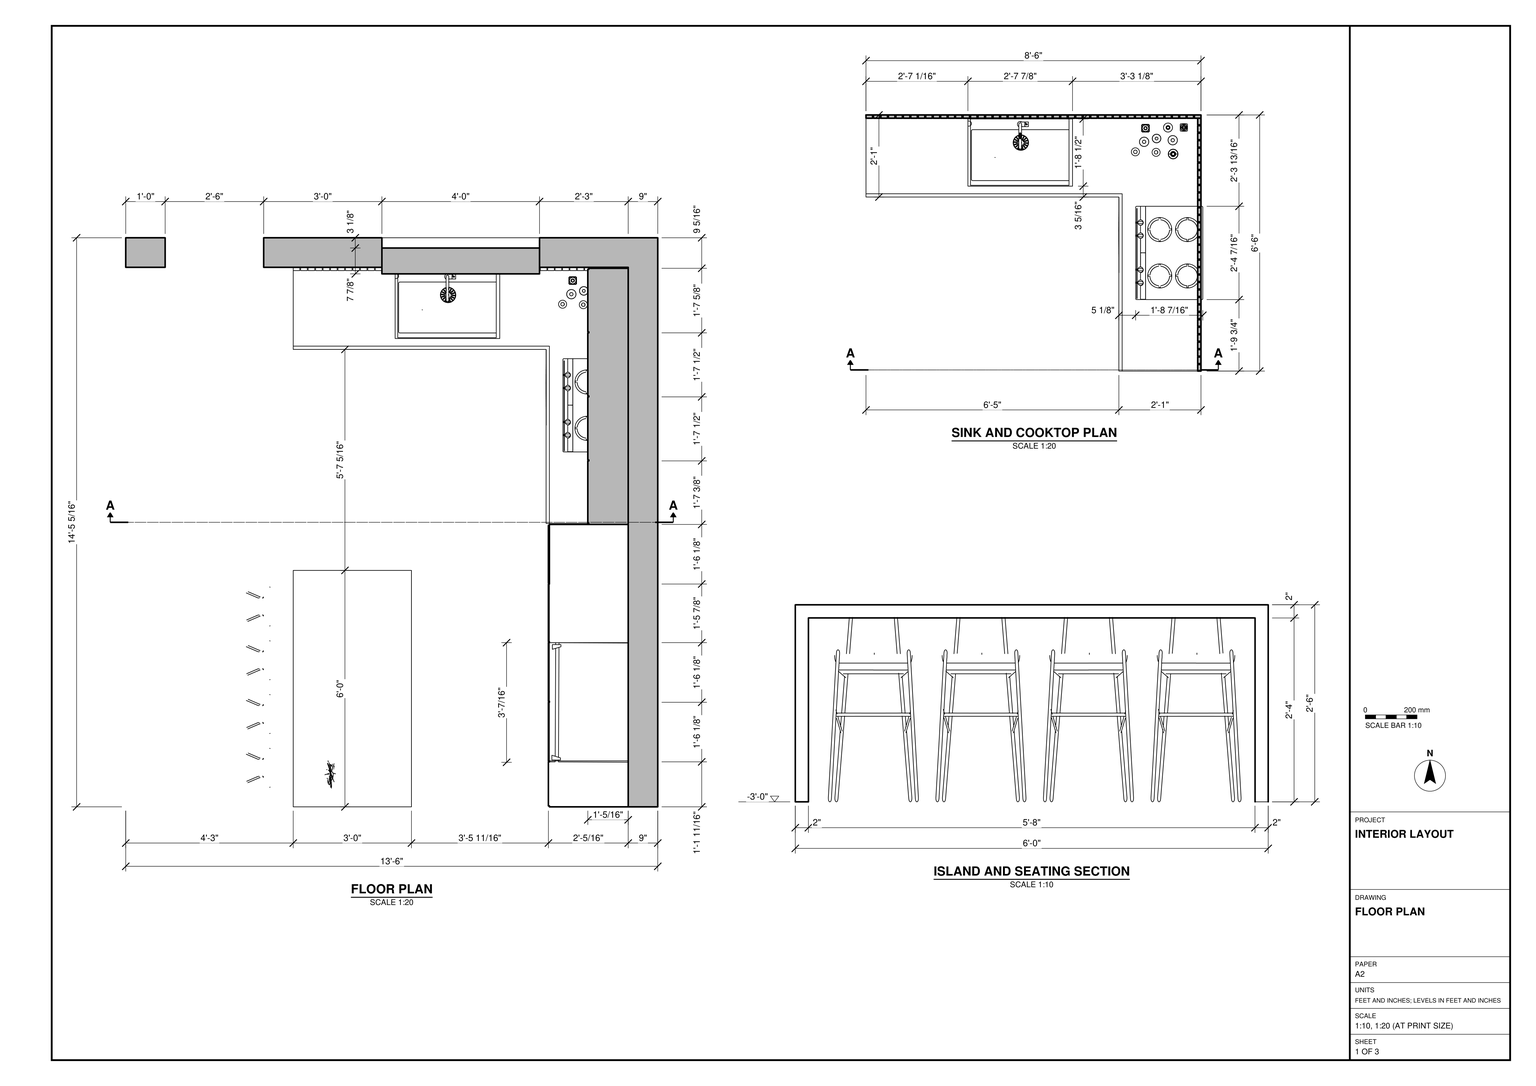
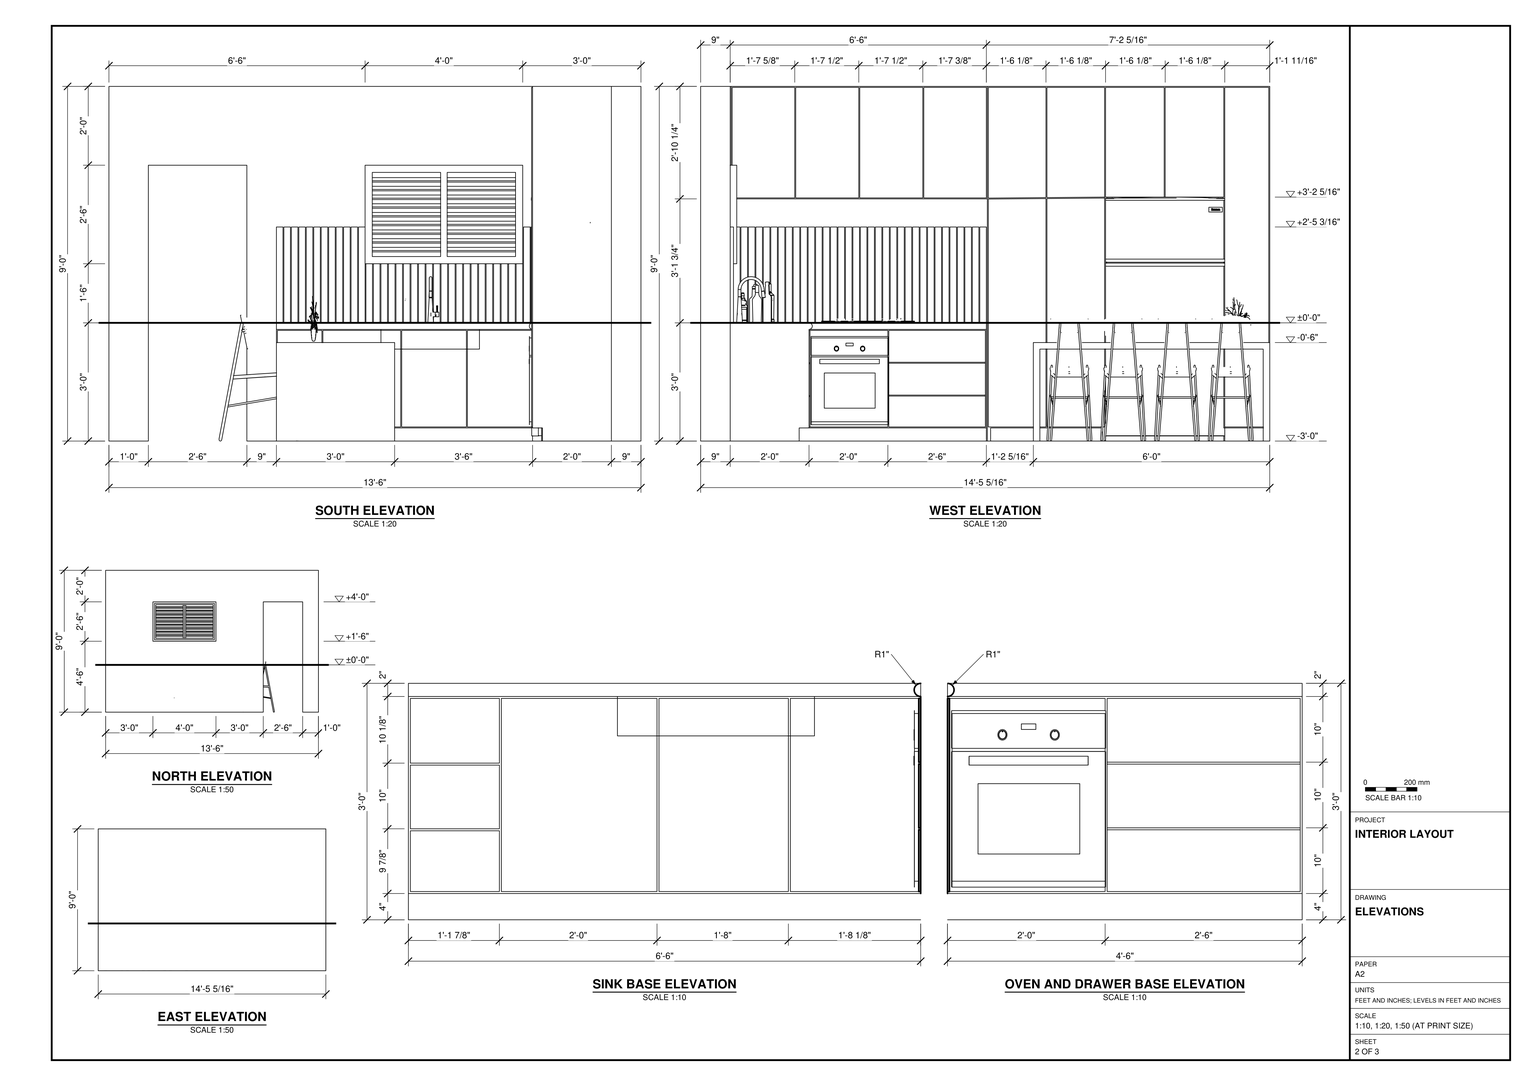
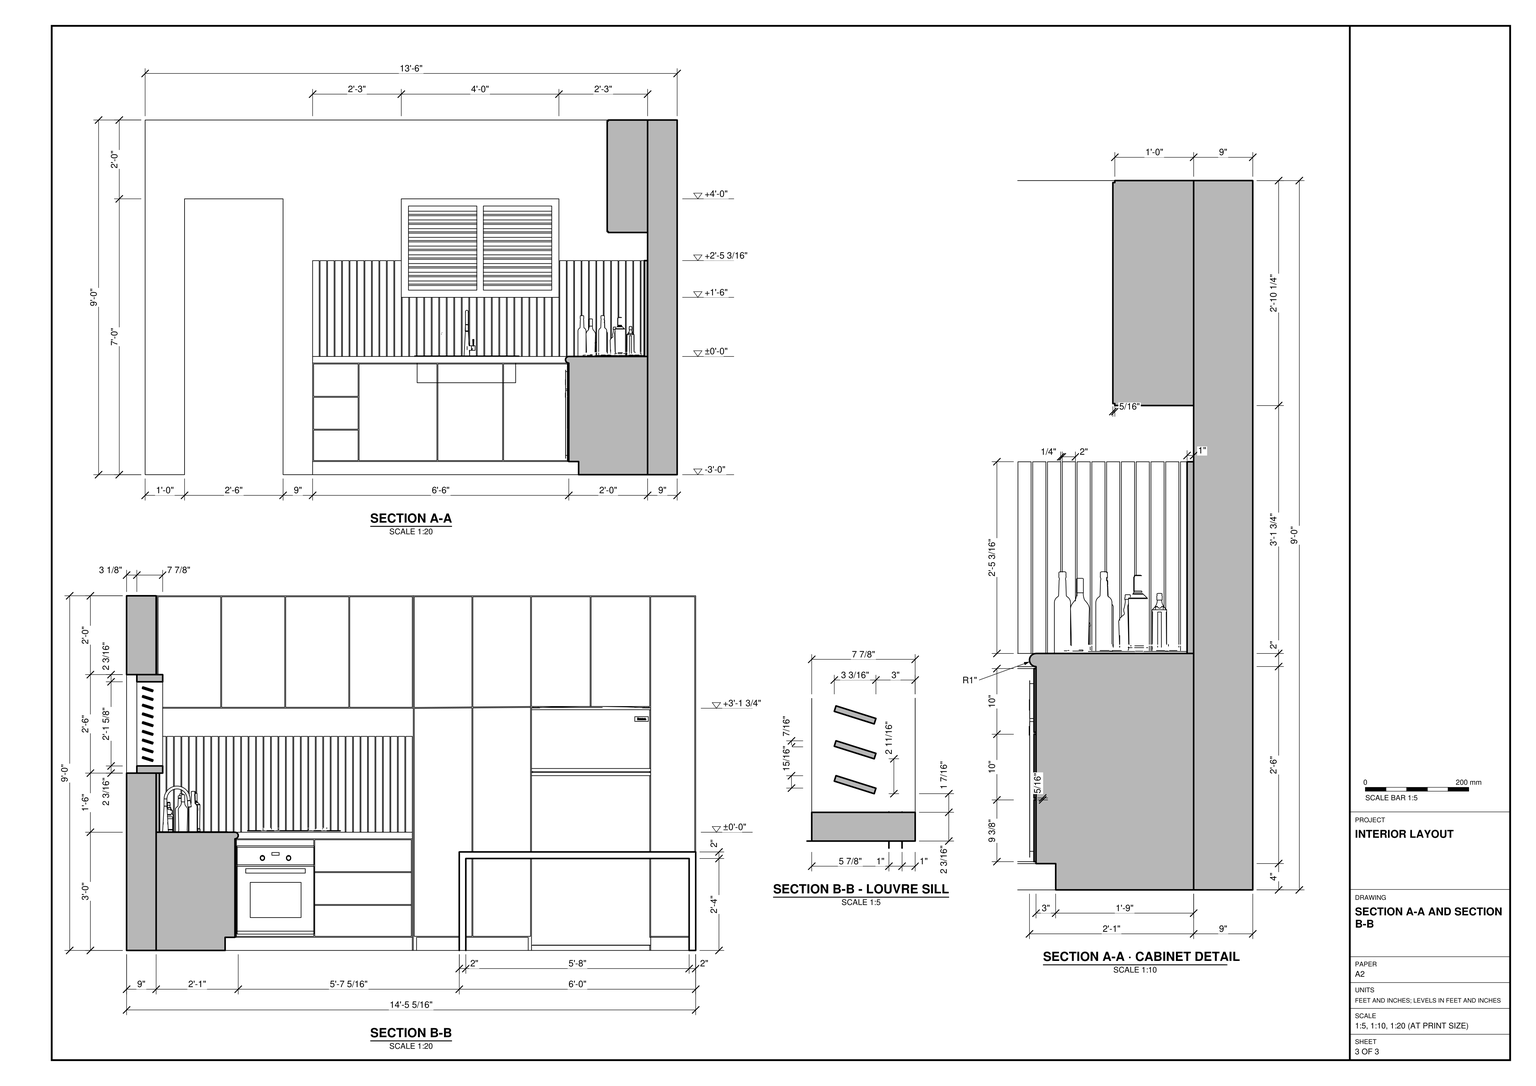
Build the kitchen in SketchUp from task_files/diagram_01.pdf. Work in feet and inches. The overall size is 13'-6" along X, 14'-5 5/16" along Y and 9'-0" high. Model a single storey at relative level ±0'-0". When reading the elevations and sections, note that their local datum is the perimeter worktop, 3'-0" above the floor.

Follow the floor plan for the wall lengths, thicknesses and openings. Leave the doorway open and set the two-panel louvred window above the sink, with its sill and angled blades as shown in section. Form the L-shaped worktop with the sink on the window wall and the cooktop on the return, above the oven. Use the cabinet elevations and details to set out the doors, drawer stacks, recessed plinths and rounded worktop edge. Include the vertically divided backsplash, the overhead cabinets and the tall storage and refrigerator bays along the return wall.

Place the freestanding island parallel to the long cabinet wall. Give it a 6'-0" by 3'-0" top, slab ends and the open underside shown in the seating section. Arrange four seats along its outer long edge, leaving the aisle between the island and the cabinets clear. Decor, loose items and appliances may be any suitable library components placed as shown.

Keep the walls and other shell elements, each furniture piece and each joinery unit in separate groups or components, and use components for repeated parts. Save one SketchUp model as output_files/kitchen_with_l_shaped_cabinetry_and_a_seating_island.skp.

# SketchUp Ruby script. Lengths in inches.
U = 1.inch
M = Sketchup.active_model
def pt(a) = Geom::Point3d.new(a.map { |v| v * U })
def face(e, loops, mat)
  f = e.add_face(loops[0].map { |a| pt(a) })
  loops[1..].each { |l| e.add_face(l.map { |a| pt(a) }).erase! }
  f.material = f.back_material = mat if mat
  f
end
# faces: each face lists its corners as indices into pts; further lists are holes
def faces(e, pts, list, mat = nil) = list.each { |f| face(e, (f[0].is_a?(Array) ? f : [f]).map { |l| l.map { |i| pts[i] } }, mat) }
# xy, xz, yz: faces in a plane at the given z, y or x. An outline is a flat list of corners, or four numbers for a rectangle; further outlines are holes
def ring(l) = l.size == 4 ? [[l[0], l[1]], [l[2], l[1]], [l[2], l[3]], [l[0], l[3]]] : l.each_slice(2).to_a
def flat(e, list, mat, &to3) = list.each { |f| face(e, (f[0].is_a?(Array) ? f : [f]).map { |l| ring(l).map { |u, v| to3.(u, v) } }, mat) }
def xy(e, z, list, mat = nil) = flat(e, list, mat) { |x, y| [x, y, z] }
def xz(e, y, list, mat = nil) = flat(e, list, mat) { |x, z| [x, y, z] }
def yz(e, x, list, mat = nil) = flat(e, list, mat) { |y, z| [x, y, z] }
def lines(e, pts, list) = list.each { |a, b| e.add_line(pt(pts[a]), pt(pts[b])) }
# prism: a flat outline (further loops are holes) pulled along v
def prism(e, loops, v, mat = nil)
  f = face(e, loops, mat); d = Geom::Vector3d.new(v.map { |x| x * U })
  f.pushpull(f.normal.samedirection?(d) ? d.length : -d.length)
end
def box(e, o, s, mat = nil) = prism(e, [[o, [o[0] + s[0], o[1], o[2]], [o[0] + s[0], o[1] + s[1], o[2]], [o[0], o[1] + s[1], o[2]]]], [0, 0, s[2]], mat)
def at(x, y, z, deg = 0) = Geom::Transformation.translation(pt([x, y, z])) * Geom::Transformation.rotation(ORIGIN, Z_AXIS, deg.degrees)
def axes(o, x, y, z) = Geom::Transformation.new([*x, 0, *y, 0, *z, 0, *pt(o).to_a, 1])
def part(name) = M.definitions.add(name)
# library, detail: a bought-in or finely detailed component or shape, given as its bounding box
def library(name, o, s) = part(name).tap { |d| box(d.entities, o, s) }
def detail(e, o, s) = box(e.add_group.entities, o, s)
def put(e, d, t, mat = nil) = e.add_instance(d, t).tap { |i| i.material = mat if mat }
def group(e, t, mat = nil) = e.add_group.tap { |g| g.transformation = t; g.material = mat if mat }.entities
root = M.entities
M.materials.add("[Color C02]").color = [255, 204, 153]
M.materials.add("[Color E08]").color = [102, 102, 0]
c1 = part("Cabinet rail")
prism(c1.entities,[[[0,0.08,0],[0,3.12,0.96],[45.8125,3.12,0.96],[45.8125,0.08,0]]],[0,-0.13,0.42])
c2 = part("Cabinet stile")
box(c2.entities,[0,0,0],[2,1,29.1875])
c3 = library("Float Chair Alt",[-11.76,1.28,-24.8],[23.52,26.7,30.06])
c4 = library("ENERGISK+B18+S (1)",[50,0,0],[28,31.125,68.4])
c5 = library("sink",[-18.39,0,-10.63],[31.85,20.47,24.5])
c6 = library("5\#1",[-14.24,-10.22,0],[28.4,20.44,1.42])
c7 = library("Группа\#24",[0,0,-0.39],[23.46,23.54,23.41])
c8 = part("духовой шкаф")
p = [[285.71,355.65,85.04],[285.71,355.46,84.84]]
lines(c8.entities,p,[[0,1]])
put(c8.entities,c7,at(-5.375,42.92,31.74))
c9 = library("plant",[0,0,0],[28.86,24.45,26.45])
c10 = library("Small Bar",[-21.2,3.96,5.71],[39.1,35.8,37.57])
c11 = part("Group17\#1")
p = [[-46.8125,-1.1875,0],[-1.1875,-1.1875,0],[-1.1875,-28.8125,0],[-46.8125,-28.8125,0]]
lines(c11.entities,p,[[0,1],[1,2],[2,3],[3,0]])
c12 = part("Group16\#1")
xy(c12.entities,0,[[[-48,-30,0,0],[-45.8125,-27.8125,-2.1875,-2.1875]],[-25,-27.8125,-24,-2.1875],[-24,-27.8125,-23,-2.1875]])
xy(c12.entities,7.875,[[[-48,-30,0,0],[-45.8125,-27.8125,-25,-2.1875],[-23,-27.8125,-2.1875,-2.1875]]])
xz(c12.entities,-30,[[-48,0,0,7.875]])
xz(c12.entities,-27.8125,[[-45.8125,0,-25,7.875],[-23,0,-2.1875,7.875]])
xz(c12.entities,-2.1875,[[-45.8125,0,-25,7.875],[-23,0,-2.1875,7.875]])
xz(c12.entities,0,[[-48,0,0,7.875]])
yz(c12.entities,-48,[[-30,0,0,7.875]])
yz(c12.entities,-45.8125,[[-27.8125,0,-2.1875,7.875]])
yz(c12.entities,-25,[[-27.8125,0,-2.1875,7.875]])
yz(c12.entities,-23,[[-27.8125,0,-2.1875,7.875]])
yz(c12.entities,-2.1875,[[-27.8125,0,-2.1875,7.875]])
yz(c12.entities,0,[[-30,0,0,7.875]])
p = [[-24,-2.1875,7.875],[-24,-2.1875,0]]
lines(c12.entities,p,[[0,1]])
put(c12.entities,c11,at(0,0,0))
c13 = part("Group\#8")
box(c13.entities,[0,0,0],[2,1,18])
c14 = part("Group\#9")
box(c14.entities,[0,0,0],[1,2,29.1875])
put(root,c1,at(80.1875,165.34,78.86))
put(root,c1,at(80.1875,165.34,76.2))
put(root,c1,at(80.1875,165.34,73.54))
put(root,c1,at(80.1875,165.34,70.89))
put(root,c1,at(80.1875,165.34,68.23))
put(root,c1,at(80.1875,165.34,65.57))
put(root,c1,at(80.1875,165.34,62.92))
put(root,c1,at(80.1875,165.34,60.26))
put(root,c1,at(80.1875,165.34,57.61))
put(root,c2,at(51,163.3,36),"[Color E08]")
put(root,c2,at(53.27,163.3,36),"[Color E08]")
put(root,c2,at(55.55,163.3,36),"[Color E08]")
put(root,c2,at(57.82,163.3,36),"[Color E08]")
put(root,c2,at(60.09,163.3,36),"[Color E08]")
put(root,c2,at(62.36,163.3,36),"[Color E08]")
put(root,c2,at(64.64,163.3,36),"[Color E08]")
put(root,c2,at(66.91,163.3,36),"[Color E08]")
put(root,c2,at(69.18,163.3,36),"[Color E08]")
put(root,c2,at(71.45,163.3,36),"[Color E08]")
put(root,c2,at(73.73,163.3,36),"[Color E08]")
put(root,c2,at(76,163.3,36),"[Color E08]")
put(root,c2,at(126.25,163.3,36),"[Color E08]")
put(root,c2,at(128.5,163.3,36),"[Color E08]")
put(root,c2,at(130.75,163.3,36),"[Color E08]")
put(root,c2,at(133,163.3,36),"[Color E08]")
put(root,c2,at(135.25,163.3,36),"[Color E08]")
put(root,c2,at(137.5,163.3,36),"[Color E08]")
put(root,c2,at(139.75,163.3,36),"[Color E08]")
put(root,c2,at(142,163.3,36),"[Color E08]")
put(root,c2,at(144.25,163.3,36),"[Color E08]")
put(root,c2,at(146.5,163.3,36),"[Color E08]")
put(root,c2,at(148.75,163.3,36),"[Color E08]")
put(root,c2,at(151,163.3,36),"[Color E08]")
put(root,c3,axes([62.34,61.01,31.64],[0,0.58351,0],[-1.03,0,0],[0,0,1.27612]))
put(root,c3,axes([62.34,44.64,31.64],[0,0.58351,0],[-1.03,0,0],[0,0,1.27612]))
put(root,c3,axes([62.34,28.26,31.64],[0,0.58351,0],[-1.03,0,0],[0,0,1.27612]))
put(root,c3,axes([62.34,11.89,31.64],[0,0.58351,0],[-1.03,0,0],[0,0,1.27612]))
put(root,c4,axes([129.07,114.82,0],[-0.00579,-1.29645,0],[1.00703,-0.0045,0],[0,0,1.08618]))
put(root,c5,at(100.42,142.61,36.2))
put(root,c6,at(143.34,122.32,36,90))
put(root,c8,axes([125.4,134.31,-31.03],[0,-1,0],[0.05952,0,0],[0,0,1.1484]))
put(root,c9,axes([63.9,5.64,30.42],[-0.11466,0,0],[0,0.34872,0],[0,0,0.52]))
put(root,c10,at(130.99,146.94,5.17))
g1 = group(root,at(51,86.3,0))
xy(g1,0,[[81,0,81,57,0,57,0,78,102,78,102,0]])
xy(g1,4,[[78,0,81,57],[0,54,78,57]])
xy(g1,28,[[31.82,54,61.82,56.6875],[31.82,56.6875,61.82,77]])
xy(g1,34,[[31.82,54,61.82,56.5625],[31.82,56.5625,61.82,56.6875]])
xy(g1,36,[[[78,0,102,0,102,78,0,78,0,54,78,54],[31.82,56.5625,61.82,77]]])
xz(g1,0,[[81,0,102,0,102,36,78,36,77.74,35.97,77.5,35.87,77.29,35.71,77.13,35.5,77.03,35.26,77,35,77.03,34.74,77.13,34.5,77.29,34.29,77.5,34.13,77.74,34.03,78,34,78,4,81,4]])
xz(g1,54,[[0,4,78,4,78,34,61.82,34,61.82,28,31.82,28,31.82,34,0,34],[78,34,77.74,34.03,77.5,34.13,77.29,34.29,77.13,34.5,77.03,34.74,77,35,77.03,35.26,77.13,35.5,77.29,35.71,77.5,35.87,77.74,35.97,78,36]])
xz(g1,56.5625,[[31.82,34,61.82,36]])
xz(g1,56.6875,[[31.82,28,61.82,34]])
xz(g1,57,[[0,0,81,4]],"[Color C02]")
xz(g1,77,[[31.82,28,61.82,36]])
xz(g1,78,[[0,0,102,36]])
yz(g1,0,[[57,0,57,4,54,4,54,34,53.74,34.03,53.5,34.13,53.29,34.29,53.13,34.5,53.03,34.74,53,35,53.03,35.26,53.13,35.5,53.29,35.71,53.5,35.87,53.74,35.97,54,36,78,36,78,0]],"[Color C02]")
yz(g1,31.82,[[54,28,56.6875,34],[56.6875,28,77,28,77,36,56.5625,36,56.5625,34,56.6875,34]])
yz(g1,61.82,[[54,28,56.6875,34],[56.6875,28,56.6875,34,56.5625,34,56.5625,36,77,36,77,28]])
yz(g1,78,[[0,4,54,34]])
yz(g1,81,[[0,0,57,4]],"[Color C02]")
yz(g1,102,[[0,0,78,36]])
p = [[77.74,0,34.03],[77.5,0,34.13],[77.5,53.5,34.13],[77.5,54,34.13],[77.74,54,34.03],[77.74,53.74,34.03],
  [78,0,34],[78,54,34],[0,53.5,34.13],[0,53.74,34.03],[78,53.74,34.03],[78,53.5,34.13],
  [0,54,34],[31.82,54,34],[61.82,54,34],[77.29,0,34.29],[77.29,53.29,34.29],[77.29,54,34.29],
  [0,53.29,34.29],[78,53.29,34.29],[77.13,0,34.5],[77.13,53.13,34.5],[77.13,54,34.5],[0,53.13,34.5],
  [78,53.13,34.5],[77.03,0,34.74],[77.03,53.03,34.74],[77.03,54,34.74],[0,53.03,34.74],[78,53.03,34.74],
  [77,0,35],[77,53,35],[77,54,35],[0,53,35],[78,53,35],[77.03,0,35.26],
  [77.03,53.03,35.26],[77.03,54,35.26],[0,53.03,35.26],[78,53.03,35.26],[77.13,0,35.5],[77.13,53.13,35.5],
  [77.13,54,35.5],[0,53.13,35.5],[78,53.13,35.5],[77.29,0,35.71],[77.29,53.29,35.71],[77.29,54,35.71],
  [0,53.29,35.71],[78,53.29,35.71],[77.5,0,35.87],[77.5,53.5,35.87],[77.5,54,35.87],[0,53.5,35.87],
  [78,53.5,35.87],[77.74,0,35.97],[77.74,53.74,35.97],[77.74,54,35.97],[0,53.74,35.97],[78,53.74,35.97],
  [78,0,36],[78,54,36],[0,54,36]]
faces(g1,p,[[0,1,2,3,4,5],[6,0,5,4,7],[8,9,5,10,11,2],[9,12,13,14,7,10,5],[1,15,16,17,3,2],[18,8,2,11,19,16],[15,20,21,22,17,16],[23,18,16,19,24,21],
  [20,25,26,27,22,21],[28,23,21,24,29,26],[25,30,31,32,27,26],[33,28,26,29,34,31],[30,35,36,37,32,31],[38,33,31,34,39,36],[35,40,41,42,37,36],[43,38,36,39,44,41],
  [40,45,46,47,42,41],[48,43,41,44,49,46],[45,50,51,52,47,46],[53,48,46,49,54,51],[50,55,56,57,52,51],[58,53,51,54,59,56],[55,60,61,57,56],[62,58,56,59,61]],"[Color C02]")
g2 = group(root,at(51.3,140.3,4),"[Color C02]")
box(g2,[57.85,-0.3,0.3],[19.55,0.3,29.4])
box(g2,[13.85,-0.3,0.3],[23.7,0.3,29.4])
box(g2,[37.85,-0.3,0.3],[19.7,0.3,29.4])
box(g2,[0,-0.3,19.85],[13.55,0.3,9.85])
box(g2,[0,-0.3,9.85],[13.55,0.3,9.7])
box(g2,[0,-0.3,0.3],[13.55,0.3,9.25])
p = [[57.85,0,30],[57.55,0,30]]
lines(g2,p,[[0,1]])
g3 = group(root,at(129,86.6,4.3),"[Color C02]")
box(g3,[-0.3,29.7,0],[0.3,23.7,29.4])
xy(g3,0,[[-0.3,0,0,29.4]])
xy(g3,9.4,[[-0.3,0,0,29.4]])
xy(g3,9.7,[[-0.3,0,0,29.4]])
xy(g3,19.4,[[-0.3,0,0,29.4]])
xy(g3,19.7,[[-0.3,0,0,29.4]])
xy(g3,29.4,[[-0.3,0,0,29.4]])
xz(g3,0,[[-0.3,0,0,9.4],[-0.3,9.7,0,19.4],[-0.3,19.7,0,29.4]])
xz(g3,29.4,[[-0.3,0,0,9.4],[-0.3,9.7,0,19.4],[-0.3,19.7,0,29.4]])
yz(g3,-0.3,[[0,0,29.4,9.4],[0,9.7,29.4,19.4],[0,19.7,29.4,29.4]])
yz(g3,0,[[0,0,29.4,9.4],[0,9.4,29.4,9.7],[0,9.7,29.4,19.4],[0,19.4,29.4,19.7],[0,19.7,29.4,29.4]])
g4 = group(root,at(128.7,0,0),"[Color C02]")
xy(g4,0,[[3.3,0,24.3,14],[0.3,50,3.3,51],[3.3,50,24.3,86],[0.3,85,3.3,86]])
xy(g4,4,[[0.3,0,3.3,14],[0.3,51,3.3,85]])
xy(g4,4.3,[[0,0.3,0.3,13.7],[0,50.3,0.3,67.85]])
xy(g4,74,[[0.3,14,24.3,50]])
xy(g4,74.3,[[0,14,0.3,31.85],[0,32.15,0.3,50]])
xy(g4,107.7,[[0,0.3,0.3,13.7],[0,14,0.3,31.85],[0,32.15,0.3,50],[0,50.3,0.3,67.85],[0,68.15,0.3,85.7]])
xy(g4,108,[[0.3,0,24.3,14],[0.3,14,24.3,50],[0.3,50,24.3,86]])
xz(g4,0,[[3.3,0,24.3,0,24.3,108,0.3,108,0.3,4,3.3,4]])
xz(g4,0.3,[[0,4.3,0.3,107.7]])
xz(g4,13.7,[[0,4.3,0.3,107.7]])
xz(g4,14,[[3.3,0,3.3,4,0.3,4,0.3,74,24.3,74,24.3,0],[0,74.3,0.3,107.7]])
xz(g4,31.85,[[0,74.3,0.3,107.7]])
xz(g4,32.15,[[0,74.3,0.3,107.7]])
xz(g4,50,[[0.3,0,24.3,74],[0,74.3,0.3,107.7]])
xz(g4,50.3,[[0,4.3,0.3,74],[0,74.3,0.3,107.7]])
xz(g4,51,[[0.3,0,3.3,4]])
xz(g4,67.85,[[0,4.3,0.3,73.85],[0,74.15,0.3,107.7]])
xz(g4,85,[[0.3,0,3.3,4]])
xz(g4,86,[[0.3,0,24.3,108]])
yz(g4,0,[[0.3,4.3,13.7,107.7],[50.3,4.3,50.3,74,67.85,73.85,67.85,4.3],[68.15,4.3,68.15,73.85,85.7,73.7,85.7,4.3],[85.7,74,68.15,74.15,68.15,107.7,85.7,107.7],[67.85,74.15,50.3,74.3,50.3,107.7,67.85,107.7],
  [14,74.3,31.85,107.7],[32.15,74.3,50,107.7]])
yz(g4,0.3,[[[50,0,50,74,14,74,14,4,0,4,0,108,86,108,86,0,85,0,85,4,51,4,51,0],[50.3,4.3,67.85,4.3,67.85,73.85,50.3,74,50.3,74.3,67.85,74.15,67.85,107.7,50.3,107.7],[0.3,4.3,13.7,107.7],[32.15,74.3,50,107.7],[14,74.3,31.85,107.7]]])
yz(g4,3.3,[[0,0,14,4],[51,0,85,4]])
yz(g4,24.3,[[0,0,14,108],[50,0,86,108],[14,74,50,108]])
p = [[0,67.85,73.85],[0,50.3,74],[0.3,50.3,74],[0.3,67.85,73.85],[0,50.3,74.3],[0,67.85,74.15],
  [0.3,67.85,74.15],[0.3,50.3,74.3]]
faces(g4,p,[[0,1,2,3],[4,5,6,7]])
g5 = group(root,at(140.7,86,73.75),"[Color C02]")
xy(g5,0,[[0.3,0,12.3,78]])
xy(g5,0.3,[[0,0.3,0.3,19.35],[0,19.65,0.3,38.85],[0,39.15,0.3,58.35],[0,58.65,0.3,77.7]])
xy(g5,33.95,[[0,0.3,0.3,19.35],[0,19.65,0.3,38.85],[0,39.15,0.3,58.35],[0,58.65,0.3,77.7]])
xy(g5,34.25,[[0.3,0,12.3,78]])
xz(g5,0,[[0.3,0,12.3,34.25]])
xz(g5,0.3,[[0,0.3,0.3,33.95]])
xz(g5,19.35,[[0,0.3,0.3,33.95]])
xz(g5,19.65,[[0,0.3,0.3,33.95]])
xz(g5,38.85,[[0,0.3,0.3,33.95]])
xz(g5,39.15,[[0,0.3,0.3,33.95]])
xz(g5,58.35,[[0,0.3,0.3,33.95]])
xz(g5,58.65,[[0,0.3,0.3,33.95]])
xz(g5,77.7,[[0,0.3,0.3,33.95]])
xz(g5,78,[[0.3,0,12.3,34.25]])
yz(g5,0,[[0.3,0.3,19.35,33.95],[19.65,0.3,38.85,33.95],[39.15,0.3,58.35,33.95],[58.65,0.3,77.7,33.95]])
yz(g5,0.3,[[[0,0,78,34.25],[39.15,0.3,58.35,33.95],[19.65,0.3,38.85,33.95],[58.65,0.3,77.7,33.95],[0.3,0.3,19.35,33.95]]])
yz(g5,12.3,[[0,0,78,34.25]])
g6 = group(root,at(51,0,0))
xy(g6,0,[[0,0,36,2]])
xy(g6,28,[[0,2,36,70]])
xy(g6,30,[[0,0,36,72]])
xz(g6,0,[[0,0,36,30]])
xz(g6,2,[[0,0,36,28]])
xz(g6,70,[[0,0,36,28]])
xz(g6,72,[[0,0,36,30]])
yz(g6,0,[[0,0,0,30,72,30,72,0,70,0,70,28,2,28,2,0]])
yz(g6,36,[[0,0,2,0,2,28,70,28,70,0,72,0,72,30,0,30]])
g7 = group(root,at(0,0,0))
xy(g7,0,[[153,0,153,164.3,42,164.3,42,173.3,162,173.3,162,0],[0,164.3,12,173.3]])
xy(g7,54,[[78,164.3,126,173.3]])
xy(g7,84,[[12,164.3,42,173.3],[78,164.3,126,173.3]])
xy(g7,108,[[153,0,162,0,162,173.3,0,173.3,0,164.3,153,164.3]])
xz(g7,0,[[153,0,162,108]])
xz(g7,164.3,[[[0,0,12,0,12,84,42,84,42,0,153,0,153,108,0,108],[78,54,126,84]]])
xz(g7,173.3,[[[0,0,0,108,162,108,162,0,42,0,42,84,12,84,12,0],[78,54,126,84]]])
yz(g7,0,[[164.3,0,173.3,108]])
yz(g7,12,[[164.3,0,173.3,84]])
yz(g7,42,[[164.3,0,173.3,84]])
yz(g7,78,[[164.3,54,173.3,84]])
yz(g7,126,[[164.3,54,173.3,84]])
yz(g7,153,[[0,0,164.3,108]])
yz(g7,162,[[0,0,173.3,108]])
put(root,c12,axes([126,170.18,84],[1,0,0],[0,0,1],[0,-1,0]))
put(root,c13,at(78.25,163.3,36),"[Color E08]")
put(root,c13,at(80.54,163.3,36),"[Color E08]")
put(root,c13,at(82.82,163.3,36),"[Color E08]")
put(root,c13,at(85.11,163.3,36),"[Color E08]")
put(root,c13,at(87.4,163.3,36),"[Color E08]")
put(root,c13,at(89.6875,163.3,36),"[Color E08]")
put(root,c13,at(91.98,163.3,36),"[Color E08]")
put(root,c13,at(94.26,163.3,36),"[Color E08]")
put(root,c13,at(96.55,163.3,36),"[Color E08]")
put(root,c13,at(98.84,163.3,36),"[Color E08]")
put(root,c13,at(101.125,163.3,36),"[Color E08]")
put(root,c13,at(103.41,163.3,36),"[Color E08]")
put(root,c13,at(105.7,163.3,36),"[Color E08]")
put(root,c13,at(107.99,163.3,36),"[Color E08]")
put(root,c13,at(110.28,163.3,36),"[Color E08]")
put(root,c13,at(112.5625,163.3,36),"[Color E08]")
put(root,c13,at(114.85,163.3,36),"[Color E08]")
put(root,c13,at(117.14,163.3,36),"[Color E08]")
put(root,c13,at(119.43,163.3,36),"[Color E08]")
put(root,c13,at(121.71,163.3,36),"[Color E08]")
put(root,c13,at(124,163.3,36),"[Color E08]")
put(root,c14,at(152,161.3,36),"[Color E08]")
put(root,c14,at(152,159.03,36),"[Color E08]")
put(root,c14,at(152,156.75,36),"[Color E08]")
put(root,c14,at(152,154.48,36),"[Color E08]")
put(root,c14,at(152,152.21,36),"[Color E08]")
put(root,c14,at(152,149.9375,36),"[Color E08]")
put(root,c14,at(152,147.66,36),"[Color E08]")
put(root,c14,at(152,145.39,36),"[Color E08]")
put(root,c14,at(152,143.12,36),"[Color E08]")
put(root,c14,at(152,140.85,36),"[Color E08]")
put(root,c14,at(152,138.57,36),"[Color E08]")
put(root,c14,at(152,136.3,36),"[Color E08]")
put(root,c14,at(152,134.03,36),"[Color E08]")
put(root,c14,at(152,131.75,36),"[Color E08]")
put(root,c14,at(152,129.48,36),"[Color E08]")
put(root,c14,at(152,127.21,36),"[Color E08]")
put(root,c14,at(152,124.9375,36),"[Color E08]")
put(root,c14,at(152,122.66,36),"[Color E08]")
put(root,c14,at(152,120.39,36),"[Color E08]")
put(root,c14,at(152,118.12,36),"[Color E08]")
put(root,c14,at(152,115.85,36),"[Color E08]")
put(root,c14,at(152,113.57,36),"[Color E08]")
put(root,c14,at(152,111.3,36),"[Color E08]")
put(root,c14,at(152,109.03,36),"[Color E08]")
put(root,c14,at(152,106.75,36),"[Color E08]")
put(root,c14,at(152,104.48,36),"[Color E08]")
put(root,c14,at(152,102.21,36),"[Color E08]")
put(root,c14,at(152,99.9375,36),"[Color E08]")
put(root,c14,at(152,97.66,36),"[Color E08]")
put(root,c14,at(152,95.39,36),"[Color E08]")
put(root,c14,at(152,93.12,36),"[Color E08]")
put(root,c14,at(152,90.85,36),"[Color E08]")
put(root,c14,at(152,88.57,36),"[Color E08]")
put(root,c14,at(152,86.3,36),"[Color E08]")
